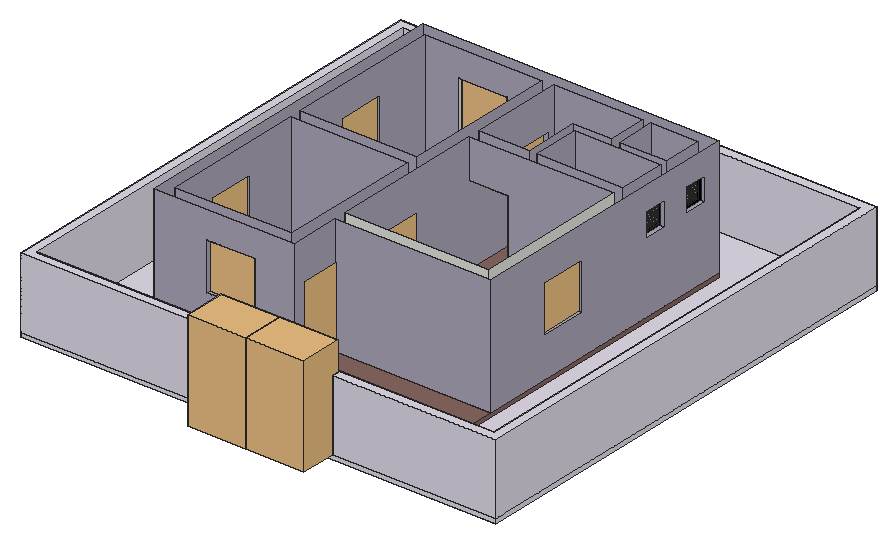
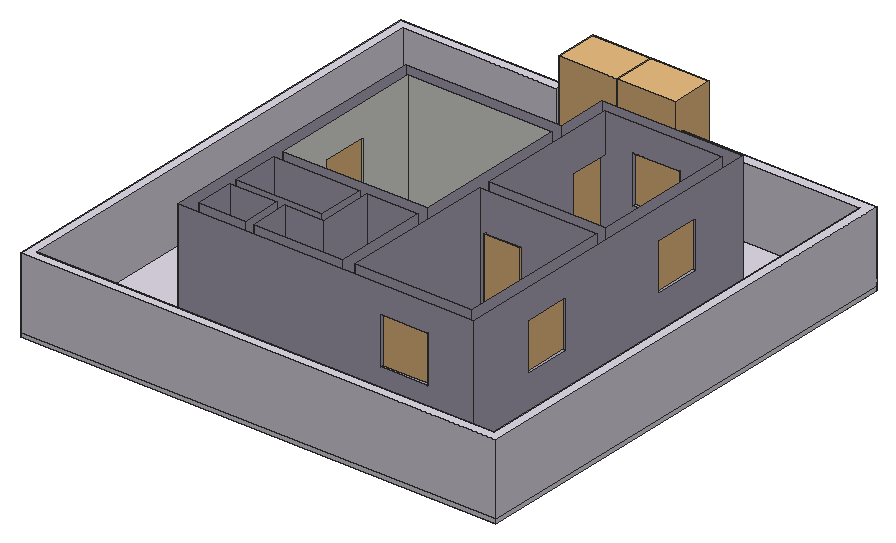
# SketchUp Ruby script. Lengths in millimetres.
U = 1.mm
M = Sketchup.active_model
def pt(a) = Geom::Point3d.new(a.map { |v| v * U })
def face(e, loops, mat)
  f = e.add_face(loops[0].map { |a| pt(a) })
  loops[1..].each { |l| e.add_face(l.map { |a| pt(a) }).erase! }
  f.material = f.back_material = mat if mat
  f
end
# faces: each face lists its corners as indices into pts; further lists are holes
def faces(e, pts, list, mat = nil) = list.each { |f| face(e, (f[0].is_a?(Array) ? f : [f]).map { |l| l.map { |i| pts[i] } }, mat) }
# xy, xz, yz: faces in a plane at the given z, y or x. An outline is a flat list of corners, or four numbers for a rectangle; further outlines are holes
def ring(l) = l.size == 4 ? [[l[0], l[1]], [l[2], l[1]], [l[2], l[3]], [l[0], l[3]]] : l.each_slice(2).to_a
def flat(e, list, mat, &to3) = list.each { |f| face(e, (f[0].is_a?(Array) ? f : [f]).map { |l| ring(l).map { |u, v| to3.(u, v) } }, mat) }
def xy(e, z, list, mat = nil) = flat(e, list, mat) { |x, y| [x, y, z] }
def xz(e, y, list, mat = nil) = flat(e, list, mat) { |x, z| [x, y, z] }
def yz(e, x, list, mat = nil) = flat(e, list, mat) { |y, z| [x, y, z] }
def lines(e, pts, list) = list.each { |a, b| e.add_line(pt(pts[a]), pt(pts[b])) }
# prism: a flat outline (further loops are holes) pulled along v
def prism(e, loops, v, mat = nil)
  f = face(e, loops, mat); d = Geom::Vector3d.new(v.map { |x| x * U })
  f.pushpull(f.normal.samedirection?(d) ? d.length : -d.length)
end
def box(e, o, s, mat = nil) = prism(e, [[o, [o[0] + s[0], o[1], o[2]], [o[0] + s[0], o[1] + s[1], o[2]], [o[0], o[1] + s[1], o[2]]]], [0, 0, s[2]], mat)
def at(x, y, z, deg = 0) = Geom::Transformation.translation(pt([x, y, z])) * Geom::Transformation.rotation(ORIGIN, Z_AXIS, deg.degrees)
def axes(o, x, y, z) = Geom::Transformation.new([*x, 0, *y, 0, *z, 0, *pt(o).to_a, 1])
def part(name) = M.definitions.add(name)
# library, detail: a bought-in or finely detailed component or shape, given as its bounding box
def library(name, o, s) = part(name).tap { |d| box(d.entities, o, s) }
def detail(e, o, s) = box(e.add_group.entities, o, s)
def put(e, d, t, mat = nil) = e.add_instance(d, t).tap { |i| i.material = mat if mat }
def group(e, t, mat = nil) = e.add_group.tap { |g| g.transformation = t; g.material = mat if mat }.entities
root = M.entities
M.materials.add("0268 AP 7144 ITALIAN IRIS").color = [172, 166, 184]
M.materials.add("0282 AP 9628 Fading Light-N").color = [223, 218, 231]
M.materials.add("[0137_Black]").color = [0, 0, 0]
M.materials.add("[Tile Mosaic Multi]").color = [135, 103, 96]
M.materials.add("[Translucent Glass Blue]").color = [100, 149, 237]
M.materials["[Translucent Glass Blue]"].alpha = 0.5
M.materials.add("[Wood Veneer 01]").color = [120, 70, 37]
c1 = library("Ornamental gate leaf",[0,0,0],[4100,1077.8,7119.6])
c2 = part("cong")
put(c2.entities,c1,axes([6217.3,5957.9,0],[-1,0,0],[0,1,0],[0,0,1]))
put(c2.entities,c1,at(6217.3,5957.9,0))
c3 = library("PINTU 6 YA",[0,-17.5,0],[910.1,205,2050])
c4 = part("Group\#2")
xy(c4.entities,0,[[0,0,300,500]])
p = [[200,500,0],[200,454.5,0],[200,409.1,0],[200,363.6,0],[200,318.2,0],[200,272.7,0],
  [200,227.3,0],[200,181.8,0],[200,136.4,0],[200,90.9,0],[200,45.5,0],[200,0,0],
  [100,45.5,0],[100,0,0],[100,500,0],[100,454.5,0],[100,318.2,0],[100,272.7,0],
  [100,227.3,0],[100,181.8,0],[100,136.4,0],[100,90.9,0],[100,409.1,0],[100,363.6,0]]
lines(c4.entities,p,[[0,1],[2,3],[4,5],[6,7],[8,9],[10,11],[12,13],[14,15],[16,17],[18,19],[20,21],[22,23]])
c5 = part("Group21\#2")
xy(c5.entities,0,[[-545.5,-545.5,-201.8,545.5],[-171.8,-545.5,171.8,545.5],[201.8,-545.5,545.5,545.5]])
c6 = part("Group20\#1")
detail(c6.entities,[-609.5,-609.5,0],[1219,1219,127])
put(c6.entities,c5,at(0,0,63.5),"[Translucent Glass Blue]")
c7 = part("Group17\#2")
xy(c7.entities,0,[[-545.5,-545.5,-201.8,545.5],[-171.8,-545.5,171.8,545.5],[201.8,-545.5,545.5,545.5]])
c8 = part("Group16\#1")
detail(c8.entities,[-609.5,-609.5,0],[1219,1219,127])
put(c8.entities,c7,at(0,0,63.5),"[Translucent Glass Blue]")
c9 = part("Group15\#2")
xy(c9.entities,0,[[-546,-546,-202,546],[-172,-546,172,546],[202,-546,546,546]])
c10 = part("Group14\#1")
detail(c10.entities,[-609.5,-609.5,0],[1219,1219,127])
put(c10.entities,c9,at(0,0,63.5),"[Translucent Glass Blue]")
c11 = part("Group19\#2")
xy(c11.entities,0,[[-545.5,-545.5,-15,545.5],[15,-545.5,545.5,545.5]])
c12 = part("Group18\#1")
detail(c12.entities,[-609.5,-609.5,0],[1219,1219,127])
put(c12.entities,c11,at(0,0,63.5),"[Translucent Glass Blue]")
c13 = part("Group23\#2")
xy(c13.entities,0,[[-545.5,-545.5,-15,545.5],[15,-545.5,545.5,545.5]])
c14 = part("Group22\#1")
detail(c14.entities,[-609.5,-609.5,0],[1219,1219,127])
put(c14.entities,c13,at(0,0,63.5),"[Translucent Glass Blue]")
c15 = part("Group27\#1")
prism(c15.entities,[[[254.2,-249.2,76.2],[254.2,-254.2,76.2],[254.2,-210.2,0],[254.2,-205.2,0]]],[-508.4,0,0])
c16 = part("Group28\#1")
prism(c16.entities,[[[254.2,-141.7,0],[254.2,-185.7,76.2],[254.2,-190.7,76.2],[254.2,-146.7,0]]],[-508.4,0,0])
c17 = part("Group29\#1")
prism(c17.entities,[[[-254.2,-78.2,0],[-254.2,-83.2,0],[-254.2,-127.2,76.2],[-254.2,-122.2,76.2]]],[508.4,0,0])
c18 = part("Group30\#1")
prism(c18.entities,[[[254.2,-63.7,76.2],[254.2,-19.7,0],[254.2,-14.7,0],[254.2,-58.7,76.2]]],[-508.4,0,0])
c19 = part("Group31\#1")
prism(c19.entities,[[[254.2,-0.2,76.2],[254.2,43.8,0],[254.2,48.8,0],[254.2,4.8,76.2]]],[-508.4,0,0])
c20 = part("Group32\#1")
prism(c20.entities,[[[254.2,68.3,76.2],[254.2,63.3,76.2],[254.2,107.3,0],[254.2,112.3,0]]],[-508.4,0,0])
c21 = part("Group33\#1")
prism(c21.entities,[[[254.2,126.8,76.2],[254.2,170.8,0],[254.2,175.8,0],[254.2,131.8,76.2]]],[-508.4,0,0])
c22 = part("Group34\#1")
prism(c22.entities,[[[254.2,190.3,76.2],[254.2,234.3,0],[254.2,239.3,0],[254.2,195.3,76.2]]],[-508.4,0,0])
c23 = part("Group35\#1")
xy(c23.entities,76.2,[[-254.2,253.8,254.2,254.2]])
p = [[254.2,253.8,76.2],[-254.2,253.8,76.2],[-254.2,254.2,75.5],[254.2,254.2,75.5]]
faces(c23.entities,p,[[0,1,2,3]])
c24 = part("Group25\#1")
put(c24.entities,c15,at(0,0,0))
put(c24.entities,c16,at(0,0,0))
put(c24.entities,c17,at(0,0,0))
put(c24.entities,c18,at(0,0,0))
put(c24.entities,c19,at(0,0,0))
put(c24.entities,c20,at(0,0,0))
put(c24.entities,c21,at(0,0,0))
put(c24.entities,c22,at(0,0,0))
put(c24.entities,c23,at(0,0,0))
c25 = part("Group38\#1")
prism(c25.entities,[[[254.2,-254.2,76],[254.2,-210.3,0],[254.2,-205.3,0],[254.2,-249.2,76]]],[-508.4,0,0])
c26 = part("Group39\#1")
prism(c26.entities,[[[-254.2,-146.3,0],[-254.2,-190.2,76],[-254.2,-185.2,76],[-254.2,-141.3,0]]],[508.4,0,0])
c27 = part("Group40\#1")
prism(c27.entities,[[[254.2,-82.3,0],[254.2,-77.3,0],[254.2,-121.2,76],[254.2,-126.2,76]]],[-508.4,0,0])
c28 = part("Group41\#1")
prism(c28.entities,[[[254.2,-13.3,0],[254.2,-57.2,76],[254.2,-62.2,76],[254.2,-18.3,0]]],[-508.4,0,0])
c29 = part("Group42\#1")
prism(c29.entities,[[[-254.2,45.7,0],[-254.2,1.8,76],[-254.2,6.8,76],[-254.2,50.7,0]]],[508.4,0,0])
c30 = part("Group43\#1")
prism(c30.entities,[[[-254.2,70.8,76],[-254.2,114.7,0],[-254.2,109.7,0],[-254.2,65.8,76]]],[508.4,0,0])
c31 = part("Group44\#1")
prism(c31.entities,[[[254.2,129.8,76],[254.2,173.7,0],[254.2,178.7,0],[254.2,134.8,76]]],[-508.4,0,0])
c32 = part("Group45\#1")
prism(c32.entities,[[[254.2,193.8,76],[254.2,237.7,0],[254.2,242.7,0],[254.2,198.8,76]]],[-508.4,0,0])
c33 = part("Group36\#1")
put(c33.entities,c25,at(0,0,0))
put(c33.entities,c26,at(0,0,0))
put(c33.entities,c27,at(0,0,0))
put(c33.entities,c28,at(0,0,0))
put(c33.entities,c29,at(0,0,0))
put(c33.entities,c30,at(0,0,0))
put(c33.entities,c31,at(0,0,0))
put(c33.entities,c32,at(0,0,0))
box(root,[0,0,-101.6],[12192,12192,101.6],"0282 AP 9628 Fading Light-N")
xy(root,101.6,[[1913.3,1897,1913.3,10497,9513.3,10497,9513.3,3197,5213.3,3197,5213.3,4847,5513.3,4847,5513.3,3497,9213.3,3497,9213.3,7497,6513.3,7497,6513.3,7797,6813.3,7797,6813.3,9197,7013.3,9197,7013.3,7797,9213.3,7797,9213.3,8997,7813.3,8997,7813.3,9297,8013.3,9297,8013.3,9197,9213.3,9197,9213.3,10197,8013.3,10197,8013.3,10097,7813.3,10097,7813.3,10197,5513.3,10197,5513.3,10047,5213.3,10047,5213.3,10197,2213.3,10197,2213.3,6197,4163.3,6197,4163.3,5897,2213.3,5897,2213.3,2197,5513.3,2197,5513.3,1897],[5213.3,5747,5513.3,9147],[5063.3,5897,5213.3,6197]])
xy(root,1123,[[9213.3,4897,9363.3,6116]])
xy(root,1123,[[9363.3,4897,9513.3,6116]],"0268 AP 7144 ITALIAN IRIS")
xy(root,1166.9,[[1913.3,7550.9,2063.3,8769.9],[2063.3,7550.9,2213.3,8769.9]],"0268 AP 7144 ITALIAN IRIS")
xy(root,1170,[[1913.3,3377.3,2063.3,4596.3],[2063.3,3377.3,2213.3,4596.3]],"0268 AP 7144 ITALIAN IRIS")
xy(root,1234.2,[[3094.3,10197,4313.3,10347]])
xy(root,1234.2,[[3094.3,10347,4313.3,10497]],"0268 AP 7144 ITALIAN IRIS")
xy(root,1238.4,[[3274.2,1897,4493.2,2047],[3274.2,2047,4493.2,2197]],"0268 AP 7144 ITALIAN IRIS")
xy(root,1930.4,[[9213.3,8147,9363.3,8757],[9363.3,8147,9513.3,8757],[9213.3,9447,9363.3,10057],[9363.3,9447,9513.3,10057]],"0268 AP 7144 ITALIAN IRIS")
xy(root,2149.6,[[5213.3,4847,5513.3,5747],[4163.3,5897,5063.3,6197],[5513.3,7497,6513.3,7797],[7013.3,8997,7813.3,9197],[5213.3,9147,5513.3,10047],
  [7813.3,9297,8013.3,10097]])
xy(root,2149.6,[[5213.3,2197,5513.3,3197]],"0268 AP 7144 ITALIAN IRIS")
xy(root,2342,[[9213.3,4897,9363.3,6116]])
xy(root,2342,[[9363.3,4897,9513.3,6116]],"0268 AP 7144 ITALIAN IRIS")
xy(root,2385.9,[[2063.3,7550.9,2213.3,8769.9]])
xy(root,2385.9,[[1913.3,7550.9,2063.3,8769.9]],"0268 AP 7144 ITALIAN IRIS")
xy(root,2389,[[2063.3,3377.3,2213.3,4596.3]])
xy(root,2389,[[1913.3,3377.3,2063.3,4596.3]],"0268 AP 7144 ITALIAN IRIS")
xy(root,2453.2,[[3094.3,10197,4313.3,10347],[3094.3,10347,4313.3,10497]])
xy(root,2457.4,[[3274.2,2047,4493.2,2197]])
xy(root,2457.4,[[3274.2,1897,4493.2,2047]],"0268 AP 7144 ITALIAN IRIS")
xy(root,2540.4,[[9213.3,8147,9363.3,8757],[9213.3,9447,9363.3,10057]])
xy(root,2540.4,[[9363.3,8147,9513.3,8757],[9363.3,9447,9513.3,10057]],"0268 AP 7144 ITALIAN IRIS")
xz(root,1897,[[[1913.3,101.6,5513.3,3149.6],[3274.2,1238.4,4493.2,2457.4]]],"0268 AP 7144 ITALIAN IRIS")
xz(root,2197,[[[2213.3,101.6,2213.3,3149.6,5213.3,3149.6,5213.3,2149.6,5513.3,2149.6,5513.3,101.6],[3274.2,1238.4,4493.2,2457.4]]],"0268 AP 7144 ITALIAN IRIS")
xz(root,3197,[[5213.3,101.6,9513.3,101.6,9513.3,3149.6,5513.3,3149.6,5513.3,2149.6,5213.3,2149.6]],"0268 AP 7144 ITALIAN IRIS")
xz(root,3377.3,[[1913.3,1170,2063.3,2389],[2063.3,1170,2213.3,2389]],"0268 AP 7144 ITALIAN IRIS")
xz(root,3497,[[5513.3,101.6,9213.3,3149.6]])
xz(root,4596.3,[[1913.3,1170,2063.3,2389],[2063.3,1170,2213.3,2389]],"0268 AP 7144 ITALIAN IRIS")
xz(root,4847,[[5213.3,101.6,5513.3,2149.6]],"0268 AP 7144 ITALIAN IRIS")
xz(root,4897,[[9213.3,1123,9363.3,2342]])
xz(root,4897,[[9363.3,1123,9513.3,2342]],"0268 AP 7144 ITALIAN IRIS")
xz(root,5747,[[5213.3,101.6,5513.3,2149.6]],"0268 AP 7144 ITALIAN IRIS")
xz(root,5897,[[2213.3,101.6,4163.3,101.6,4163.3,2149.6,5063.3,2149.6,5063.3,101.6,5213.3,101.6,5213.3,3149.6,2213.3,3149.6]],"0268 AP 7144 ITALIAN IRIS")
xz(root,6116,[[9213.3,1123,9363.3,2342]])
xz(root,6116,[[9363.3,1123,9513.3,2342]],"0268 AP 7144 ITALIAN IRIS")
xz(root,6197,[[2213.3,101.6,2213.3,3149.6,5213.3,3149.6,5213.3,101.6,5063.3,101.6,5063.3,2149.6,4163.3,2149.6,4163.3,101.6]],"0268 AP 7144 ITALIAN IRIS")
xz(root,7497,[[6513.3,101.6,9213.3,101.6,9213.3,3149.6,5513.3,3149.6,5513.3,2149.6,6513.3,2149.6]],"0268 AP 7144 ITALIAN IRIS")
xz(root,7550.9,[[1913.3,1166.9,2063.3,2385.9],[2063.3,1166.9,2213.3,2385.9]],"0268 AP 7144 ITALIAN IRIS")
xz(root,7797,[[6513.3,101.6,6513.3,2149.6,5513.3,2149.6,5513.3,3149.6,6813.3,3149.6,6813.3,101.6],[7013.3,101.6,9213.3,3149.6]],"0268 AP 7144 ITALIAN IRIS")
xz(root,8147,[[9213.3,1930.4,9363.3,2540.4],[9363.3,1930.4,9513.3,2540.4]],"0268 AP 7144 ITALIAN IRIS")
xz(root,8757,[[9213.3,1930.4,9363.3,2540.4],[9363.3,1930.4,9513.3,2540.4]],"0268 AP 7144 ITALIAN IRIS")
xz(root,8769.9,[[1913.3,1166.9,2063.3,2385.9],[2063.3,1166.9,2213.3,2385.9]],"0268 AP 7144 ITALIAN IRIS")
xz(root,8997,[[7813.3,101.6,9213.3,101.6,9213.3,3149.6,7013.3,3149.6,7013.3,2149.6,7813.3,2149.6]],"0268 AP 7144 ITALIAN IRIS")
xz(root,9147,[[5213.3,101.6,5513.3,2149.6]],"0268 AP 7144 ITALIAN IRIS")
xz(root,9197,[[6813.3,101.6,6813.3,3149.6,7813.3,3149.6,7813.3,2149.6,7013.3,2149.6,7013.3,101.6],[8013.3,101.6,9213.3,3149.6]],"0268 AP 7144 ITALIAN IRIS")
xz(root,9297,[[7813.3,101.6,8013.3,2149.6]],"0268 AP 7144 ITALIAN IRIS")
xz(root,9447,[[9213.3,1930.4,9363.3,2540.4],[9363.3,1930.4,9513.3,2540.4]],"0268 AP 7144 ITALIAN IRIS")
xz(root,10047,[[5213.3,101.6,5513.3,2149.6]],"0268 AP 7144 ITALIAN IRIS")
xz(root,10057,[[9213.3,1930.4,9363.3,2540.4],[9363.3,1930.4,9513.3,2540.4]],"0268 AP 7144 ITALIAN IRIS")
xz(root,10097,[[7813.3,101.6,8013.3,2149.6]],"0268 AP 7144 ITALIAN IRIS")
xz(root,10197,[[[2213.3,101.6,5213.3,3149.6],[3094.3,1234.2,4313.3,2453.2]],[5513.3,101.6,7813.3,3149.6],[8013.3,101.6,9213.3,3149.6]],"0268 AP 7144 ITALIAN IRIS")
xz(root,10497,[[[1913.3,101.6,9513.3,3149.6],[3094.3,1234.2,4313.3,2453.2]]],"0268 AP 7144 ITALIAN IRIS")
yz(root,1913.3,[[[1897,101.6,10497,3149.6],[3377.3,1170,4596.3,2389],[7550.9,1166.9,8769.9,2385.9]]],"0268 AP 7144 ITALIAN IRIS")
yz(root,2213.3,[[[2197,101.6,5897,3149.6],[3377.3,1170,4596.3,2389]],[[6197,101.6,10197,3149.6],[7550.9,1166.9,8769.9,2385.9]]],"0268 AP 7144 ITALIAN IRIS")
yz(root,3094.3,[[10197,1234.2,10347,2453.2]])
yz(root,3094.3,[[10347,1234.2,10497,2453.2]],"0268 AP 7144 ITALIAN IRIS")
yz(root,3274.2,[[1897,1238.4,2047,2457.4],[2047,1238.4,2197,2457.4]],"0268 AP 7144 ITALIAN IRIS")
yz(root,4163.3,[[5897,101.6,6197,2149.6]],"0268 AP 7144 ITALIAN IRIS")
yz(root,4313.3,[[10197,1234.2,10347,2453.2]])
yz(root,4313.3,[[10347,1234.2,10497,2453.2]],"0268 AP 7144 ITALIAN IRIS")
yz(root,4493.2,[[1897,1238.4,2047,2457.4],[2047,1238.4,2197,2457.4]],"0268 AP 7144 ITALIAN IRIS")
yz(root,5063.3,[[5897,101.6,6197,2149.6]],"0268 AP 7144 ITALIAN IRIS")
yz(root,5213.3,[[3197,101.6,3197,2149.6,2197,2149.6,2197,3149.6,5897,3149.6,5897,101.6,5747,101.6,5747,2149.6,4847,2149.6,4847,101.6],[6197,101.6,6197,3149.6,10197,3149.6,10197,101.6,10047,101.6,10047,2149.6,9147,2149.6,9147,101.6]],"0268 AP 7144 ITALIAN IRIS")
yz(root,5513.3,[[1897,101.6,2197,101.6,2197,2149.6,3197,2149.6,3197,3149.6,1897,3149.6],[3497,101.6,4847,101.6,4847,2149.6,5747,2149.6,5747,101.6,9147,101.6,9147,2149.6,10047,2149.6,10047,101.6,10197,101.6,10197,3149.6,7797,3149.6,7797,2149.6,7497,2149.6,7497,3149.6,3497,3149.6]],"0268 AP 7144 ITALIAN IRIS")
yz(root,6513.3,[[7497,101.6,7797,2149.6]],"0268 AP 7144 ITALIAN IRIS")
yz(root,6813.3,[[7797,101.6,9197,3149.6]],"0268 AP 7144 ITALIAN IRIS")
yz(root,7013.3,[[7797,101.6,9197,101.6,9197,2149.6,8997,2149.6,8997,3149.6,7797,3149.6]],"0268 AP 7144 ITALIAN IRIS")
yz(root,7813.3,[[8997,101.6,9197,2149.6],[9197,101.6,9197,3149.6,10197,3149.6,10197,101.6,10097,101.6,10097,2149.6,9297,2149.6,9297,101.6]],"0268 AP 7144 ITALIAN IRIS")
yz(root,8013.3,[[9197,101.6,9297,101.6,9297,2149.6,10097,2149.6,10097,101.6,10197,101.6,10197,3149.6,9197,3149.6]],"0268 AP 7144 ITALIAN IRIS")
yz(root,9213.3,[[[3497,101.6,7497,3149.6],[4897,1123,6116,2342]]])
yz(root,9213.3,[[[7797,101.6,8997,3149.6],[8147,1930.4,8757,2540.4]],[[9197,101.6,10197,3149.6],[9447,1930.4,10057,2540.4]]],"0268 AP 7144 ITALIAN IRIS")
yz(root,9513.3,[[[3197,101.6,10497,3149.6],[4897,1123,6116,2342],[9447,1930.4,10057,2540.4],[8147,1930.4,8757,2540.4]]],"0268 AP 7144 ITALIAN IRIS")
p = [[9363.3,9497.8,1981.2],[9363.3,10006.2,1981.2],[9363.3,10006.2,2489.6],[9363.3,9497.8,2489.6]]
lines(root,p,[[0,1],[2,3],[1,2],[3,0]])
put(root,c2,axes([4227,-6848.7,0],[0.3648,0,0],[0,1,0],[0,0,0.36]))
g1 = group(root,at(0,0,0),"0282 AP 9628 Fading Light-N")
xy(g1,0,[[0,0,4999.4,228.6],[4999.4,0,7999.4,0,7999.4,228.6,11963.4,228.6,11963.4,11963.4,228.6,11963.4,228.6,228.6,4999.4,228.6],[7999.4,0,12192,228.6]])
xy(g1,1828.8,[[0,0,4999.4,0,4999.4,228.6,228.6,228.6,228.6,11963.4,11963.4,11963.4,11963.4,228.6,7999.4,228.6,7999.4,0,12192,0,12192,12192,0,12192]])
xz(g1,0,[[0,0,4999.4,1828.8],[7999.4,0,12192,1828.8]])
xz(g1,228.6,[[228.6,0,4999.4,1828.8],[7999.4,0,11963.4,1828.8]])
xz(g1,11963.4,[[228.6,0,11963.4,1828.8]])
xz(g1,12192,[[0,0,12192,1828.8]])
yz(g1,0,[[0,0,12192,1828.8]])
yz(g1,228.6,[[228.6,0,11963.4,1828.8]])
yz(g1,4999.4,[[0,0,228.6,1828.8]])
yz(g1,7999.4,[[0,0,228.6,1828.8]])
yz(g1,11963.4,[[228.6,0,11963.4,1828.8]])
yz(g1,12192,[[0,0,12192,1828.8]])
g2 = group(root,at(1913.3,1897,0),"[Tile Mosaic Multi]")
box(g2,[0,0,0],[7600,8600,101.6])
put(root,c3,axes([7813.3,9073.9,101.6],[-0.87025,0,0],[0,0.23049,0],[0,0,0.9999]))
put(root,c3,axes([7913.3,9305,101.6],[0,0.87025,0],[0.23049,0,0],[0,0,0.9999]))
put(root,c3,axes([5349.8,3197,101.6],[0,-1.09881,0],[1,0,0],[0,0,1]))
put(root,c3,axes([5352.9,10047,101.6],[0,-1.00034,0],[-0.14451,0,0],[0,0,1]),"0268 AP 7144 ITALIAN IRIS")
put(root,c3,axes([5363.3,4847,101.6],[0,0.98893,0],[1,0,0],[0,0,1]))
put(root,c3,axes([5063.3,6047,101.6],[-0.98893,0,0],[0,1,0],[0,0,1]))
put(root,c4,at(9213.3,8147,101.6))
put(root,c4,at(9213.3,9447,101.6))
put(root,c6,axes([9299.8,5506.5,1732.5],[0,1,0],[0,0,1],[1,0,0]),"[Wood Veneer 01]")
put(root,c8,axes([2126.8,8160.4,1776.4],[0,-1,0],[0,0,1],[-1,0,0]),"[Wood Veneer 01]")
put(root,c10,axes([2126.8,3986.8,1779.5],[0,-1,0],[0,0,1],[-1,0,0]),"[Wood Veneer 01]")
put(root,c12,axes([3703.8,10283.5,1843.7],[-1,0,0],[0,0,1],[0,1,0]),"[Wood Veneer 01]")
put(root,c14,axes([3883.7,2110.5,1847.9],[1,0,0],[0,0,1],[0,-1,0]),"[Wood Veneer 01]")
g3 = group(root,at(9363.3,8757,2540.4),"0268 AP 7144 ITALIAN IRIS")
xy(g3,-610,[[-38.1,-610,38.1,0]],"[0137_Black]")
xy(g3,-559.2,[[-38.1,-559.2,0,-50.8],[0,-559.2,38.1,-50.8]],"[0137_Black]")
xy(g3,-50.8,[[-38.1,-559.2,0,-50.8],[0,-559.2,38.1,-50.8]],"[0137_Black]")
xy(g3,0,[[-38.1,-610,38.1,0]],"[0137_Black]")
xz(g3,-610,[[-38.1,-610,38.1,0]],"[0137_Black]")
xz(g3,-559.2,[[-38.1,-559.2,0,-50.8],[0,-559.2,38.1,-50.8]],"[0137_Black]")
xz(g3,-50.8,[[-38.1,-559.2,0,-50.8],[0,-559.2,38.1,-50.8]],"[0137_Black]")
xz(g3,0,[[-38.1,-610,38.1,0]],"[0137_Black]")
yz(g3,-38.1,[[[-610,-610,0,0],[-559.2,-559.2,-50.8,-50.8]]],"[0137_Black]")
yz(g3,38.1,[[[-610,-610,0,0],[-559.2,-559.2,-50.8,-50.8]]],"[0137_Black]")
put(g3,c24,axes([-38.1,-305,-305],[0,-1,0],[0,0,-1],[1,0,0]))
g4 = group(root,at(9363.3,9447,1930.4),"[0137_Black]")
prism(g4,[[[-38.1,610,610],[-38.1,610,0],[-38.1,0,0],[-38.1,0,610]],[[-38.1,559.2,50.8],[-38.1,559.2,559.2],[-38.1,50.8,559.2],[-38.1,50.8,50.8]]],[76.2,0,0])
put(root,c33,axes([9325.3,9752,2186.1],[0,1,0],[0,0,-1],[1,0,0]),"0268 AP 7144 ITALIAN IRIS")
